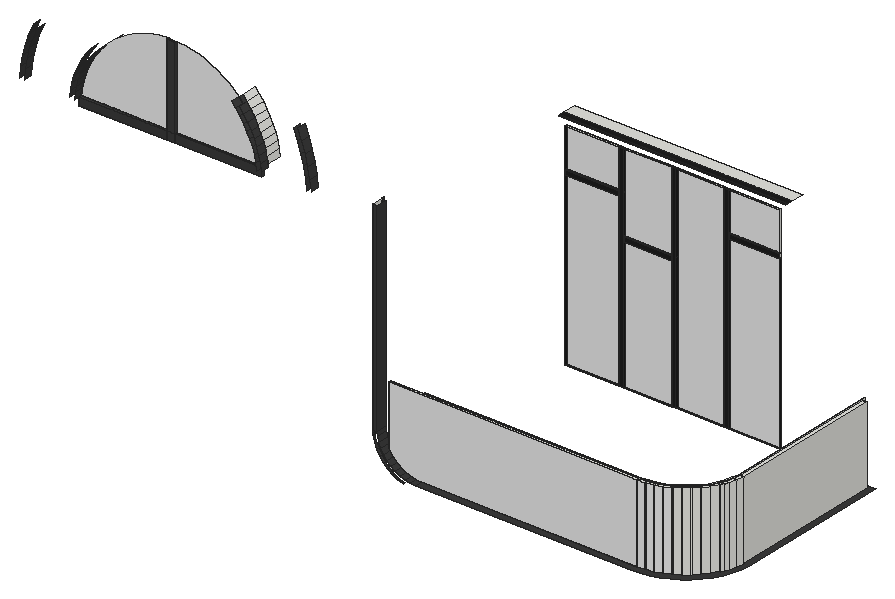
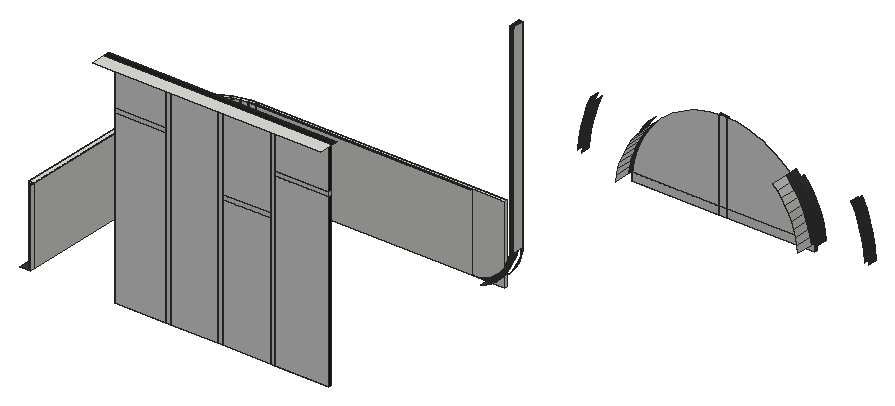
# SketchUp Ruby script. Lengths in inches.
U = 1.inch
M = Sketchup.active_model
def pt(a) = Geom::Point3d.new(a.map { |v| v * U })
def face(e, loops, mat)
  f = e.add_face(loops[0].map { |a| pt(a) })
  loops[1..].each { |l| e.add_face(l.map { |a| pt(a) }).erase! }
  f.material = f.back_material = mat if mat
  f
end
# faces: each face lists its corners as indices into pts; further lists are holes
def faces(e, pts, list, mat = nil) = list.each { |f| face(e, (f[0].is_a?(Array) ? f : [f]).map { |l| l.map { |i| pts[i] } }, mat) }
# xy, xz, yz: faces in a plane at the given z, y or x. An outline is a flat list of corners, or four numbers for a rectangle; further outlines are holes
def ring(l) = l.size == 4 ? [[l[0], l[1]], [l[2], l[1]], [l[2], l[3]], [l[0], l[3]]] : l.each_slice(2).to_a
def flat(e, list, mat, &to3) = list.each { |f| face(e, (f[0].is_a?(Array) ? f : [f]).map { |l| ring(l).map { |u, v| to3.(u, v) } }, mat) }
def xy(e, z, list, mat = nil) = flat(e, list, mat) { |x, y| [x, y, z] }
def xz(e, y, list, mat = nil) = flat(e, list, mat) { |x, z| [x, y, z] }
def yz(e, x, list, mat = nil) = flat(e, list, mat) { |y, z| [x, y, z] }
def lines(e, pts, list) = list.each { |a, b| e.add_line(pt(pts[a]), pt(pts[b])) }
# prism: a flat outline (further loops are holes) pulled along v
def prism(e, loops, v, mat = nil)
  f = face(e, loops, mat); d = Geom::Vector3d.new(v.map { |x| x * U })
  f.pushpull(f.normal.samedirection?(d) ? d.length : -d.length)
end
def box(e, o, s, mat = nil) = prism(e, [[o, [o[0] + s[0], o[1], o[2]], [o[0] + s[0], o[1] + s[1], o[2]], [o[0], o[1] + s[1], o[2]]]], [0, 0, s[2]], mat)
def at(x, y, z, deg = 0) = Geom::Transformation.translation(pt([x, y, z])) * Geom::Transformation.rotation(ORIGIN, Z_AXIS, deg.degrees)
def axes(o, x, y, z) = Geom::Transformation.new([*x, 0, *y, 0, *z, 0, *pt(o).to_a, 1])
def part(name) = M.definitions.add(name)
# library, detail: a bought-in or finely detailed component or shape, given as its bounding box
def library(name, o, s) = part(name).tap { |d| box(d.entities, o, s) }
def detail(e, o, s) = box(e.add_group.entities, o, s)
def put(e, d, t, mat = nil) = e.add_instance(d, t).tap { |i| i.material = mat if mat }
def group(e, t, mat = nil) = e.add_group.tap { |g| g.transformation = t; g.material = mat if mat }.entities
root = M.entities
M.materials.add("[Color M07]").color = [58, 58, 58]
M.materials.add("[Color M08]").color = [30, 30, 30]
M.materials.add("[Mirror 02]").color = [229, 229, 229]
xy(root,133.9375,[[330.59,3.37,330.67,3.38,330.59,4.75],[235.91,3.375,330.59,3.375,330.5,4.74,330.59,4.75,235.91,4.75],[330.59,3.375,330.5,4.74,330.59,4.75],[330.67,3.38,333.9375,3.58,333.68,4.92,333.85,4.95,330.59,4.75],[333.9375,3.57,334.11,3.6,333.85,4.95,333.9375,3.58],
  [333.9375,3.58,333.68,4.92,333.85,4.95],[334.11,3.6,337.19,4.18,336.78,5.48,336.94,5.53,333.85,4.95],[337.2,4.17,337.36,4.22,336.94,5.53,337.19,4.18],[337.19,4.18,336.78,5.48,336.94,5.53],[337.36,4.22,340.35,5.18,339.78,6.42,339.93,6.49,336.94,5.53],
  [340.36,5.17,340.51,5.24,339.93,6.49,340.35,5.18],[340.35,5.18,339.78,6.42,339.93,6.49],[340.51,5.24,343.37,6.57,342.64,7.72,342.79,7.8125,339.93,6.49],[343.37,6.56,343.52,6.65,342.79,7.8125,343.37,6.57],[343.37,6.57,342.64,7.72,342.79,7.8125],
  [343.52,6.65,346.18,8.3125,345.32,9.37,345.45,9.48,342.79,7.8125],[346.1875,8.3,346.32,8.41,345.45,9.48,346.18,8.3125],[346.18,8.3125,345.32,9.37,345.45,9.48],[346.32,8.41,348.76,10.39,347.78,11.34,347.9,11.46,345.45,9.48],[348.77,10.38,348.89,10.51,347.9,11.46,348.76,10.39],
  [348.76,10.39,347.78,11.34,347.9,11.46],[348.89,10.51,351.07,12.77,349.97,13.59,350.07,13.73,347.9,11.46],[351.07,12.77,349.97,13.59,350.07,13.73],[351.07,12.77,351.17,12.91,350.07,13.73],[351.17,12.91,353.05,15.43,351.95,16.24,350.07,13.73],
  [353.13,15.58,354.6875,18.31,353.51,18.98,351.95,16.24],[355.3,18.23,353.51,18.98,354.71,21.88,354.2,20.01,355.85,19.56],[356.07,19.5,356.58,21.37,354.71,21.88,356.5,21.14,355.85,19.56],[355.85,19.56,356.5,21.14,354.71,21.88,354.2,20.01],[356.58,21.37,357.42,24.4,355.55,24.91,354.71,21.88],
  [357.45,24.63,357.9,27.7,356,27.98,355.55,24.91],[356,27.98,357.9375,95.25]])
xy(root,133.9375,[[235.91,0,330.74,0,334.4375,0.23,338.11,0.92,341.66,2.06,345.05,3.63,348.22,5.6,351.12,7.96,353.7,10.65,355.9375,13.64,357.78,16.88,359.21,20.33,360.21,23.93,360.75,27.63,360.75,96.75,356,96.75,356,95.25,357.9375,95.25,357.9375,27.98,356,27.98,357.9,27.7,357.45,24.63,355.55,24.91,357.42,24.4,356.58,21.37,356.07,19.5,355.85,19.56,355.3,18.23,353.51,18.98,354.6875,18.31,353.13,15.58,351.95,16.24,353.05,15.43,351.17,12.91,351.07,12.77,348.89,10.51,348.77,10.38,348.76,10.39,346.32,8.41,346.1875,8.3,346.18,8.3125,343.52,6.65,343.37,6.56,343.37,6.57,340.51,5.24,340.36,5.17,340.35,5.18,337.36,4.22,337.2,4.17,337.19,4.18,334.11,3.6,333.9375,3.57,333.9375,3.58,330.67,3.38,330.59,3.37,330.59,3.375,235.91,3.375]],"[Color M07]")
xy(root,133.94,[[221.35,3.375,235.85,4.75]])
xy(root,134.95,[[247.98,96.75,249.98,97.5625],[270.98,96.75,272.98,97.5625],[293.99,96.75,295.99,97.5625]])
xy(root,134.95,[[224.36,96.75,247.98,97.5625],[249.98,96.75,270.98,97.5625],[272.98,96.75,293.99,97.5625],[295.99,96.75,318.45,97.5625]],"[Color M08]")
xy(root,149.34,[[217.25,0,219.1875,4.75]])
xy(root,168,[[330.59,3.37,330.67,3.38,330.59,4.75],[221.35,3.375,330.59,3.375,330.5,4.74,330.59,4.75,221.35,4.75],[330.59,3.375,330.59,4.75,330.5,4.74],[330.67,3.38,333.9375,3.58,333.68,4.92,333.85,4.95,330.59,4.75],[333.9375,3.57,334.11,3.6,333.85,4.95,333.9375,3.58],
  [333.9375,3.58,333.85,4.95,333.68,4.92],[334.11,3.6,337.19,4.18,336.78,5.48,336.94,5.53,333.85,4.95],[337.2,4.17,337.36,4.22,336.94,5.53,337.19,4.18],[337.19,4.18,336.94,5.53,336.78,5.48],[337.36,4.22,340.35,5.18,339.78,6.42,339.93,6.49,336.94,5.53],
  [235.85,4.75,330.59,4.75,333.85,4.95,336.94,5.53,339.93,6.49,342.79,7.8125,345.45,9.48,347.9,11.46,350.07,13.73,351.95,16.24,353.51,18.98,354.71,21.88,355.55,24.91,356,27.98,356,96.75,355.36,96.75,355.36,28.03,354.92,25.04,354.1,22.09,352.93,19.26,351.41,16.6,349.58,14.14,347.46,11.93,345.08,10,342.48,8.38,339.7,7.09,336.78,6.16,333.77,5.59,330.57,5.39,235.85,5.39],[340.36,5.17,340.51,5.24,339.93,6.49,340.35,5.18],[340.35,5.18,339.93,6.49,339.78,6.42],[340.51,5.24,343.37,6.57,342.64,7.72,342.79,7.8125,339.93,6.49],[343.37,6.56,343.52,6.65,342.79,7.8125,343.37,6.57],
  [343.37,6.57,342.79,7.8125,342.64,7.72],[343.52,6.65,346.18,8.3125,345.32,9.37,345.45,9.48,342.79,7.8125],[346.1875,8.3,346.32,8.41,345.45,9.48,346.18,8.3125],[346.18,8.3125,345.45,9.48,345.32,9.37],[346.32,8.41,348.76,10.39,347.78,11.34,347.9,11.46,345.45,9.48],
  [348.77,10.38,348.89,10.51,347.9,11.46,348.76,10.39],[348.76,10.39,347.9,11.46,347.78,11.34],[348.89,10.51,351.07,12.77,349.97,13.59,350.07,13.73,347.9,11.46],[351.07,12.77,350.07,13.73,349.97,13.59],[351.07,12.77,351.17,12.91,350.07,13.73],
  [351.17,12.91,353.05,15.43,351.95,16.24,350.07,13.73],[353.13,15.58,354.6875,18.31,353.51,18.98,351.95,16.24],[355.3,18.23,355.85,19.56,354.2,20.01,354.71,21.88,353.51,18.98],[356.07,19.5,356.58,21.37,354.71,21.88,356.5,21.14,355.85,19.56],[355.85,19.56,356.5,21.14,354.71,21.88,354.2,20.01],
  [356.58,21.37,357.42,24.4,355.55,24.91,354.71,21.88],[357.45,24.63,357.9,27.7,356,27.98,355.55,24.91],[356,27.98,357.9375,95.25]])
xy(root,192.15,[[249.98,96.75,270.98,97.5625]])
xy(root,194.15,[[249.98,96.75,270.98,97.5625]],"[Color M08]")
xy(root,209.62,[[224.36,96.75,247.98,97.5625],[295.99,96.75,318.45,97.5625]])
xy(root,211.62,[[224.36,96.75,247.98,97.5625],[295.99,96.75,318.45,97.5625]],"[Color M08]")
xy(root,212.44,[[105.32,26.6875,108.92,27.75]])
xy(root,212.44,[[66.96,26.6875,105.32,27.75],[108.92,26.6875,147,27.75]],"[Color M07]")
xy(root,216,[[105.32,26.6875,108.92,27.75]])
xy(root,216,[[66.96,26.6875,105.32,27.75],[108.92,26.6875,147,27.75]],"[Color M07]")
xy(root,229.05,[[224.36,96.75,247.98,97.5625],[247.98,96.75,249.98,97.5625],[249.98,96.75,270.98,97.5625],[270.98,96.75,272.98,97.5625],[272.98,96.75,293.99,97.5625],
  [293.99,96.75,295.99,97.5625],[295.99,96.75,318.45,97.5625]])
xy(root,232,[[221.4,99.875,321.4,105.75]])
xy(root,232,[[221.4,96.75,321.4,97.5625],[221.4,97.5625,321.4,99.875]],"[Color M08]")
xz(root,0,[[217.25,149.34,219.1875,238.1]],"[Color M07]")
xz(root,3.375,[[235.91,133.9375,330.59,133.9375,330.59,168,221.35,168,221.35,133.94,235.85,133.94]],"[Mirror 02]")
xz(root,4.75,[[235.91,133.9375,235.85,133.94,235.85,168,330.59,168,330.59,133.9375],[221.35,133.94,221.35,138.97,221.99,138.15,223.86,136.35,225.97,134.82,227.63,133.94],[235.85,133.94,233.52,134.1,231.24,134.59,229.05,135.38,227,136.47,225.11,137.84,223.43,139.45,221.99,141.28,221.35,142.39,221.35,168,235.85,168]])
xz(root,4.75,[[227.63,133.94,225.97,134.82,223.86,136.35,221.99,138.15,221.35,138.97,221.35,142.39,221.99,141.28,223.43,139.45,225.11,137.84,227,136.47,229.05,135.38,231.24,134.59,233.52,134.1,235.85,133.94],[221.35,138.97,220.38,140.19,219.08,142.44,218.09,144.85,217.46,147.37,217.25,149.24,217.25,149.34,219.1875,149.34,219.37,147.71,219.9375,145.45,220.82,143.3,221.35,142.39],[217.25,149.34,219.1875,238.1]],"[Color M07]")
xz(root,26.6875,[[66.96,212.44,105.32,216],[105.32,212.44,108.92,216],[108.92,212.44,147,216],[105.32,216,108.92,216,108.92,251.93,106.98,252,105.32,251.9375]],"[Color M07]")
xz(root,27.75,[[66.96,212.44,105.32,216],[105.32,212.44,108.92,216],[108.92,212.44,147,216],[105.32,216,105.32,251.9375,106.98,252,108.92,251.93,108.92,216]])
xz(root,27.75,[[66.96,216,105.32,216,105.32,251.9375,104.03,251.89,101.1,251.57,98.21,251.03,95.35,250.28,92.57,249.33,89.85,248.17,87.23,246.82,84.72,245.28,82.33,243.57,80.0625,241.68,77.95,239.625,75.98,237.43,74.1875,235.09,72.57,232.625,71.13,230.05,69.89,227.38,68.85,224.62,68.01,221.8,67.375,218.92],[108.92,216,147,216,146.58,218.92,145.95,221.8,145.11,224.62,144.07,227.38,142.82,230.05,141.39,232.625,139.77,235.09,137.97,237.43,136.01,239.625,133.89,241.68,131.63,243.57,129.24,245.28,126.72,246.82,124.1,248.17,121.39,249.33,118.6,250.28,115.75,251.03,112.85,251.57,109.92,251.89,108.92,251.93]],"[Mirror 02]")
xz(root,27.98,[[356,133.9375,357.9375,168]])
xz(root,95.25,[[356,133.9375,357.9375,168]])
xz(root,96.75,[[247.98,134.95,249.98,229.05],[270.98,134.95,272.98,229.05],[293.99,134.95,295.99,229.05],[249.98,192.15,270.98,194.15],[224.36,209.62,247.98,211.62],
  [295.99,209.62,318.45,211.62]],"[Color M08]")
xz(root,97.5625,[[247.98,134.95,249.98,229.05],[270.98,134.95,272.98,229.05],[293.99,134.95,295.99,229.05],[249.98,192.15,270.98,194.15],[224.36,209.62,247.98,211.62],
  [295.99,209.62,318.45,211.62]])
xz(root,97.5625,[[224.36,134.95,247.98,209.62],[249.98,134.95,270.98,192.15],[272.98,134.95,293.99,229.05],[295.99,134.95,318.45,209.62],[249.98,194.15,270.98,229.05],
  [224.36,211.62,247.98,229.05],[295.99,211.62,318.45,229.05]],"[Mirror 02]")
yz(root,66.96,[[26.6875,212.44,27.75,216]],"[Color M07]")
yz(root,105.32,[[26.6875,212.44,27.75,216]])
yz(root,105.32,[[26.6875,216,27.75,251.9375]],"[Color M07]")
yz(root,108.92,[[26.6875,212.44,27.75,216]])
yz(root,108.92,[[26.6875,216,27.75,251.93]],"[Color M07]")
yz(root,147,[[26.6875,212.44,27.75,216]],"[Color M07]")
yz(root,217.25,[[0.75,149.34,4.75,238.1]])
yz(root,217.25,[[0,149.24,0.75,149.34],[4.75,149.24,6.3,238.34],[0,149.34,0.75,238.1]],"[Color M07]")
yz(root,219.1875,[[0,149.34,4.75,238.1]],"[Color M07]")
yz(root,221.35,[[3.375,133.94,4.75,168]])
yz(root,224.36,[[96.75,209.62,97.5625,211.62]])
yz(root,224.36,[[96.75,134.95,97.5625,209.62],[96.75,211.62,97.5625,229.05]],"[Color M08]")
yz(root,247.98,[[96.75,209.62,97.5625,211.62]])
yz(root,247.98,[[96.75,134.95,97.5625,209.62],[96.75,211.62,97.5625,229.05]],"[Color M08]")
yz(root,249.98,[[96.75,192.15,97.5625,194.15]])
yz(root,249.98,[[96.75,134.95,97.5625,192.15],[96.75,194.15,97.5625,211.62],[96.75,211.62,97.5625,229.05]],"[Color M08]")
yz(root,270.98,[[96.75,192.15,97.5625,194.15]])
yz(root,270.98,[[96.75,134.95,97.5625,192.15],[96.75,194.15,97.5625,229.05]],"[Color M08]")
yz(root,272.98,[[96.75,134.95,97.5625,194.15],[96.75,194.15,97.5625,229.05]],"[Color M08]")
yz(root,293.99,[[96.75,134.95,97.5625,229.05]],"[Color M08]")
yz(root,295.99,[[96.75,209.62,97.5625,211.62]])
yz(root,295.99,[[96.75,134.95,97.5625,209.62],[96.75,211.62,97.5625,229.05]],"[Color M08]")
yz(root,318.45,[[96.75,209.62,97.5625,211.62],[96.75,211.62,97.5625,229.05]])
yz(root,318.45,[[96.75,134.95,97.5625,209.62]],"[Color M08]")
yz(root,330.59,[[3.37,133.9375,3.375,168],[3.375,133.9375,4.75,168]])
yz(root,333.9375,[[3.57,133.9375,3.58,168]])
yz(root,343.37,[[6.56,133.9375,6.57,168]])
yz(root,356,[[27.98,133.9375,95.25,168],[95.25,133.9375,96.75,168]])
yz(root,357.9375,[[27.98,133.9375,95.25,168]])
p = [[230.71,0.75,132.72],[230.71,0,132.72],[228.27,0,133.61],[228.27,0.75,133.61],[230.71,4.75,132.72],[230.71,6.3,132.72],
  [228.27,6.3,133.61],[228.27,4.75,133.61],[225.97,0,134.82],[225.97,0.75,134.82],[225.97,6.3,134.82],[225.97,4.75,134.82],
  [227.63,4.75,133.94],[235.91,0,133.9375],[235.91,3.375,133.9375],[235.85,3.375,133.94],[235.85,4.75,133.94],[233.52,4.75,134.1],
  [233.52,0,134.1],[235.91,4.75,133.9375],[330.5,4.74,133.9375],[330.59,3.375,133.9375],[330.59,3.375,168],[330.5,4.74,168],
  [330.59,4.75,133.9375],[330.59,4.75,168],[330.67,3.38,168],[330.67,3.38,133.9375],[330.59,3.37,168],[330.59,3.37,133.9375],
  [333.9375,3.58,133.9375],[333.9375,3.58,168],[333.68,4.92,133.9375],[333.68,4.92,168],[333.85,4.95,133.9375],[333.85,4.95,168],
  [334.11,3.6,168],[334.11,3.6,133.9375],[333.9375,3.57,168],[333.9375,3.57,133.9375],[337.19,4.18,133.9375],[337.19,4.18,168],
  [336.78,5.48,133.9375],[336.78,5.48,168],[336.94,5.53,133.9375],[336.94,5.53,168],[337.36,4.22,168],[337.36,4.22,133.9375],
  [337.2,4.17,168],[337.2,4.17,133.9375],[340.35,5.18,133.9375],[340.35,5.18,168],[339.78,6.42,133.9375],[339.78,6.42,168],
  [339.93,6.49,133.9375],[339.93,6.49,168],[340.51,5.24,168],[340.51,5.24,133.9375],[340.36,5.17,168],[340.36,5.17,133.9375],
  [343.37,6.57,133.9375],[343.37,6.57,168],[342.79,7.8125,168],[342.79,7.8125,133.9375],[342.64,7.72,133.9375],[342.64,7.72,168],
  [343.52,6.65,168],[343.52,6.65,133.9375],[343.37,6.56,168],[343.37,6.56,133.9375],[346.18,8.3125,133.9375],[346.18,8.3125,168],
  [345.45,9.48,168],[345.45,9.48,133.9375],[345.32,9.37,133.9375],[345.32,9.37,168],[346.32,8.41,133.9375],[346.32,8.41,168],
  [346.1875,8.3,168],[346.1875,8.3,133.9375],[348.76,10.39,133.9375],[348.76,10.39,168],[347.9,11.46,168],[347.9,11.46,133.9375],
  [347.78,11.34,133.9375],[347.78,11.34,168],[348.89,10.51,133.9375],[348.89,10.51,168],[348.77,10.38,168],[348.77,10.38,133.9375],
  [351.07,12.77,133.9375],[351.07,12.77,168],[350.07,13.73,168],[350.07,13.73,133.9375],[349.97,13.59,133.9375],[349.97,13.59,168],
  [351.17,12.91,133.9375],[351.17,12.91,168],[353.05,15.43,133.9375],[353.05,15.43,168],[351.95,16.24,168],[351.95,16.24,133.9375],
  [353.13,15.58,133.9375],[353.13,15.58,168],[354.6875,18.31,168],[354.6875,18.31,133.9375],[353.51,18.98,168],[353.51,18.98,133.9375],
  [355.3,18.23,133.9375],[355.3,18.23,168],[355.85,19.56,133.9375],[356.5,21.14,133.9375],[356.5,21.14,168],[355.85,19.56,168],
  [354.71,21.88,168],[354.71,21.88,133.9375],[354.2,20.01,168],[354.2,20.01,133.9375],[356.07,19.5,133.9375],[356.07,19.5,168],
  [356.58,21.37,133.9375],[356.58,21.37,168],[357.42,24.4,133.9375],[357.42,24.4,168],[355.55,24.91,168],[355.55,24.91,133.9375],
  [357.45,24.63,133.9375],[357.45,24.63,168],[357.9,27.7,133.9375],[357.9,27.7,168],[356,27.98,168],[356,27.98,133.9375],
  [231.24,4.75,134.59],[231.24,0,134.59],[229.05,4.75,135.38],[229.05,0,135.38],[223.86,0,136.35],[223.86,0.75,136.35],
  [223.86,6.3,136.35],[223.86,4.75,136.35],[227,4.75,136.47],[227,0,136.47],[221.99,0,138.15],[221.99,0.75,138.15],
  [221.99,6.3,138.15],[221.99,4.75,138.15],[225.11,4.75,137.84],[225.11,0,137.84],[223.43,4.75,139.45],[223.43,0,139.45],
  [220.38,0,140.19],[220.38,0.75,140.19],[220.38,6.3,140.19],[220.38,4.75,140.19],[221.35,4.75,138.97],[221.99,4.75,141.28],
  [221.99,0,141.28],[219.08,0,142.44],[219.08,0.75,142.44],[219.08,6.3,142.44],[219.08,4.75,142.44],[221.35,4.75,142.39],
  [220.82,4.75,143.3],[220.82,0,143.3],[218.09,0,144.85],[218.09,0.75,144.85],[218.09,6.3,144.85],[218.09,4.75,144.85],
  [219.9375,4.75,145.45],[219.9375,0,145.45],[217.67,0,146.52],[217.67,0.75,146.52],[217.46,6.3,147.37],[217.46,4.75,147.37],
  [219.37,4.75,147.71],[219.37,0,147.71],[217.46,0,147.37],[217.46,0.75,147.37],[217.35,0.74,148.3],[217.43,0.75,147.62],
  [217.35,0,148.3],[217.25,6.3,149.24],[217.25,4.75,149.24],[217.26,0,149.16],[217.26,0.75,149.16],[219.1875,4.75,149.34],
  [219.1875,0,149.34],[217.25,0,149.24],[217.25,0.75,149.24],[45.02,27.75,215.89],[45.49,27.75,220.52],[45.49,24.0625,220.52],
  [45.02,24.0625,215.89],[168.46,27.75,220.52],[168.94,27.75,215.89],[168.94,24.0625,215.89],[168.46,24.0625,220.52],[43.45,27.75,220.8],
  [42.96,27.75,216],[42.96,24.0625,216],[43.45,24.0625,220.8],[66.96,26.6875,216],[66.96,27.75,216],[67.375,27.75,218.92],
  [67.375,24.0625,218.92],[66.96,24.0625,216],[146.58,24.0625,218.92],[146.58,27.75,218.92],[147,27.75,216],[147,26.6875,216],
  [147,24.0625,216],[171,27.75,216],[170.51,27.75,220.8],[170.51,24.0625,220.8],[171,24.0625,216],[67.375,29.9375,218.92],
  [66.96,29.9375,216],[147,29.9375,216],[146.58,29.9375,218.92],[67.375,36.75,218.92],[66.96,36.75,216],[147,36.75,216],
  [146.58,36.75,218.92],[65.35,27.75,219.28],[64.9,27.75,216.15],[64.9,24.0625,216.15],[65.35,24.0625,219.28],[149.06,27.75,216.15],
  [148.61,27.75,219.28],[148.61,24.0625,219.28],[149.06,24.0625,216.15],[68.01,27.75,221.8],[68.01,24.0625,221.8],[145.95,24.0625,221.8],
  [145.95,27.75,221.8],[68.01,29.9375,221.8],[145.95,29.9375,221.8],[68.01,36.75,221.8],[145.95,36.75,221.8],[66.01,27.75,222.3125],
  [66.01,24.0625,222.3125],[147.95,27.75,222.3125],[147.95,24.0625,222.3125],[46.32,27.75,225.12],[46.32,24.0625,225.12],[167.64,27.75,225.12],
  [167.64,24.0625,225.12],[44.31,27.75,225.56],[44.31,24.0625,225.56],[169.65,27.75,225.56],[169.65,24.0625,225.56],[68.85,27.75,224.62],
  [68.85,24.0625,224.62],[145.11,24.0625,224.62],[145.11,27.75,224.62],[68.85,29.9375,224.62],[145.11,29.9375,224.62],[68.85,36.75,224.62],
  [145.11,36.75,224.62],[66.89,27.75,225.28],[66.89,24.0625,225.28],[147.06,27.75,225.28],[147.06,24.0625,225.28],[69.89,27.75,227.38],
  [69.89,24.0625,227.38],[144.07,24.0625,227.38],[144.07,27.75,227.38],[69.89,29.9375,227.38],[144.07,29.9375,227.38],[69.89,36.75,227.38],
  [144.07,36.75,227.38],[47.49,27.75,229.64],[47.49,24.0625,229.64],[166.47,27.75,229.64],[166.47,24.0625,229.64],[67.99,27.75,228.18],
  [67.99,24.0625,228.18],[145.97,27.75,228.18],[145.97,24.0625,228.18],[45.52,27.75,230.23],[45.52,24.0625,230.23],[168.44,27.75,230.23],
  [168.44,24.0625,230.23],[71.13,27.75,230.05],[71.13,24.0625,230.05],[142.82,24.0625,230.05],[142.82,27.75,230.05],[71.13,29.9375,230.05],
  [142.82,29.9375,230.05],[71.13,36.75,230.05],[142.82,36.75,230.05],[69.3,27.75,230.99],[69.3,24.0625,230.99],[144.66,27.75,230.99],
  [144.66,24.0625,230.99],[49,27.75,234.07],[49,24.0625,234.07],[164.96,27.75,234.07],[164.96,24.0625,234.07],[72.57,27.75,232.625],
  [72.57,24.0625,232.625],[141.39,24.0625,232.625],[141.39,27.75,232.625],[72.57,29.9375,232.625],[141.39,29.9375,232.625],[72.57,36.75,232.625],
  [141.39,36.75,232.625],[47.07,27.75,234.81],[47.07,24.0625,234.81],[166.89,27.75,234.81],[166.89,24.0625,234.81],[70.81,27.75,233.69],
  [70.81,24.0625,233.69],[143.15,27.75,233.69],[143.15,24.0625,233.69],[74.1875,27.75,235.09],[74.1875,24.0625,235.09],[139.77,24.0625,235.09],
  [139.77,27.75,235.09],[74.1875,29.9375,235.09],[139.77,29.9375,235.09],[74.1875,36.75,235.09],[139.77,36.75,235.09],[72.51,27.75,236.28],
  [72.51,24.0625,236.28],[141.45,27.75,236.28],[141.45,24.0625,236.28],[50.83,27.75,238.37],[50.83,24.0625,238.37],[163.125,27.75,238.37],
  [163.125,24.0625,238.37],[48.97,27.75,239.25],[48.97,24.0625,239.25],[164.99,27.75,239.25],[164.99,24.0625,239.25],[75.98,27.75,237.43],
  [75.98,24.0625,237.43],[137.97,24.0625,237.43],[137.97,27.75,237.43],[75.98,29.9375,237.43],[137.97,29.9375,237.43],[75.98,36.75,237.43],
  [137.97,36.75,237.43],[74.4,27.75,238.74],[74.4,24.0625,238.74],[139.5625,27.75,238.74],[139.5625,24.0625,238.74],[77.95,27.75,239.625],
  [77.95,24.0625,239.625],[136.01,24.0625,239.625],[136.01,27.75,239.625],[77.95,29.9375,239.625],[136.01,29.9375,239.625],[77.95,36.75,239.625],
  [136.01,36.75,239.625]]
faces(root,p,[[0,1,2,3],[4,5,6,7],[3,2,8,9],[7,6,10,11,12],[13,14,15,16,17,18],[18,17,132,133],[133,132,134,135],[9,8,136,137],
  [11,10,138,139],[135,134,140,141],[137,136,142,143],[139,138,144,145],[141,140,146,147],[147,146,148,149],[143,142,150,151],[145,144,152,153,154],
  [149,148,155,156],[151,150,157,158],[153,152,159,160],[156,155,161,162,163],[158,157,164,165],[160,159,166,167],[163,162,168,169],[165,164,170,171],
  [167,166,172,173],[169,168,174,175],[171,170,176,177],[178,179,177,176,180],[173,172,181,182],[183,184,179,178,180],[175,174,185,186],[187,188,184,183],
  [189,190,191,192],[193,194,195,196],[197,198,199,200],[201,202,203,204,205],[206,207,208,209,210],[211,212,213,214],[215,216,202,203],[217,218,207,208],
  [223,224,225,226],[227,228,229,230],[204,203,231,232],[233,234,207,206],[235,215,203,231],[218,236,234,207],[239,223,226,240],[228,241,242,229],
  [190,243,244,191],[245,193,196,246],[247,197,200,248],[212,249,250,213],[232,231,251,252],[253,254,234,233],[255,235,231,251],[236,256,254,234],
  [259,239,240,260],[241,261,262,242],[252,251,263,264],[265,266,254,253],[267,255,251,263],[256,268,266,254],[243,271,272,244],[273,245,246,274],
  [275,259,260,276],[261,277,278,262],[279,247,248,280],[249,281,282,250],[264,263,283,284],[285,286,266,265],[287,267,263,283],[268,288,286,266],
  [291,275,276,292],[277,293,294,278],[271,295,296,272],[297,273,274,298],[284,283,299,300],[301,302,286,285],[303,287,283,299],[288,304,302,286],
  [307,279,280,308],[281,309,310,282],[311,291,292,312],[293,313,314,294],[300,299,315,316],[317,318,302,301],[319,303,299,315],[304,320,318,302],
  [323,311,312,324],[313,325,326,314],[295,327,328,296],[329,297,298,330],[331,307,308,332],[309,333,334,310],[316,315,335,336],[337,338,318,317],
  [339,319,315,335],[320,340,338,318],[343,323,324,344],[325,345,346,326],[336,335,347,348],[349,350,338,337],[351,339,335,347],[340,352,350,338]],"[Color M07]")
faces(root,p,[[19,16,15,14],[20,21,22,23],[24,25,26,27],[27,26,28,29],[32,30,31,33],[34,35,31,30],[34,35,36,37],[37,36,38,39],
  [42,40,41,43],[44,45,41,40],[44,45,46,47],[47,46,48,49],[48,41,40,49],[25,24,20,23],[24,25,35,34],[35,34,32,33],
  [34,35,45,44],[52,50,51,53],[54,55,51,50],[54,55,56,57],[57,56,58,59],[58,51,50,59],[45,44,42,43],[44,45,55,54],
  [55,54,52,53],[54,55,62,63],[64,60,61,65],[63,62,61,60],[63,62,66,67],[67,66,68,69],[66,67,70,71],[62,63,64,65],
  [63,62,72,73],[74,70,71,75],[73,72,71,70],[76,77,78,79],[78,71,70,79],[73,72,77,76],[77,76,80,81],[72,73,74,75],
  [73,72,82,83],[84,80,81,85],[83,82,81,80],[86,87,88,89],[88,81,80,89],[83,82,87,86],[87,86,90,91],[82,83,84,85],
  [83,82,92,93],[94,90,91,95],[93,92,91,90],[96,97,91,90],[93,92,97,96],[97,96,98,99],[92,93,94,95],[93,92,100,101],
  [101,100,99,98],[100,101,102,103],[104,103,102,105],[101,100,106,107],[106,107,108,109],[109,108,110,111,112,113],[107,106,104,105],[107,106,114,115],
  [116,117,110,118,119,113],[120,121,119,118],[114,115,117,116],[115,114,112,111],[115,114,121,120],[121,120,122,123],[115,114,124,125],[125,124,123,122],
  [124,125,126,127],[127,126,128,129],[125,124,130,131],[131,130,129,128],[219,215,216,220],[221,217,218,222],[237,235,215,219],[222,218,236,238],
  [257,255,235,237],[238,236,256,258],[269,267,255,257],[258,256,268,270],[289,287,267,269],[270,268,288,290],[305,303,287,289],[290,288,304,306],
  [321,319,303,305],[306,304,320,322],[341,339,319,321],[322,320,340,342],[353,351,339,341],[342,340,352,354]])
faces(root,p,[[26,27,30,31],[36,37,40,41],[46,47,50,51],[56,57,60,61]],"[Mirror 02]")
